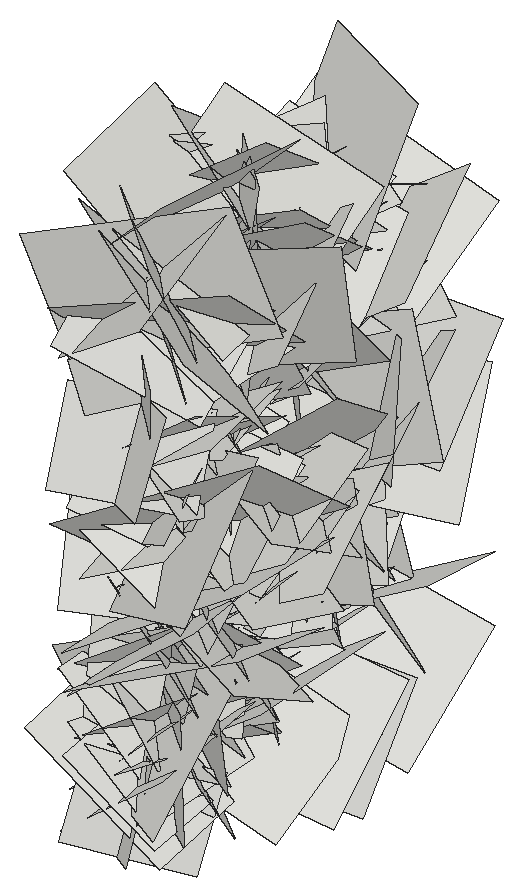
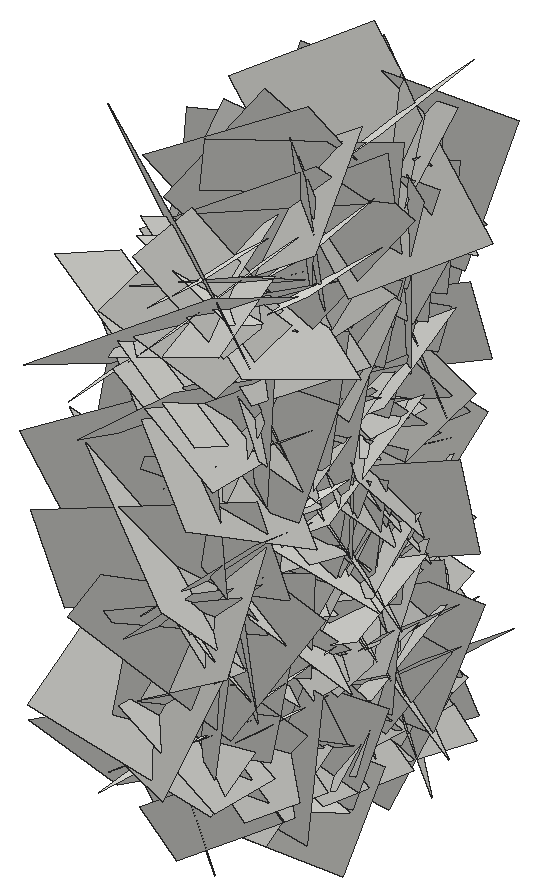
# SketchUp Ruby script. Lengths in inches.
U = 1.inch
M = Sketchup.active_model
def pt(a) = Geom::Point3d.new(a.map { |v| v * U })
def face(e, loops, mat)
  f = e.add_face(loops[0].map { |a| pt(a) })
  loops[1..].each { |l| e.add_face(l.map { |a| pt(a) }).erase! }
  f.material = f.back_material = mat if mat
  f
end
# faces: each face lists its corners as indices into pts; further lists are holes
def faces(e, pts, list, mat = nil) = list.each { |f| face(e, (f[0].is_a?(Array) ? f : [f]).map { |l| l.map { |i| pts[i] } }, mat) }
# xy, xz, yz: faces in a plane at the given z, y or x. An outline is a flat list of corners, or four numbers for a rectangle; further outlines are holes
def ring(l) = l.size == 4 ? [[l[0], l[1]], [l[2], l[1]], [l[2], l[3]], [l[0], l[3]]] : l.each_slice(2).to_a
def flat(e, list, mat, &to3) = list.each { |f| face(e, (f[0].is_a?(Array) ? f : [f]).map { |l| ring(l).map { |u, v| to3.(u, v) } }, mat) }
def xy(e, z, list, mat = nil) = flat(e, list, mat) { |x, y| [x, y, z] }
def xz(e, y, list, mat = nil) = flat(e, list, mat) { |x, z| [x, y, z] }
def yz(e, x, list, mat = nil) = flat(e, list, mat) { |y, z| [x, y, z] }
def lines(e, pts, list) = list.each { |a, b| e.add_line(pt(pts[a]), pt(pts[b])) }
# prism: a flat outline (further loops are holes) pulled along v
def prism(e, loops, v, mat = nil)
  f = face(e, loops, mat); d = Geom::Vector3d.new(v.map { |x| x * U })
  f.pushpull(f.normal.samedirection?(d) ? d.length : -d.length)
end
def box(e, o, s, mat = nil) = prism(e, [[o, [o[0] + s[0], o[1], o[2]], [o[0] + s[0], o[1] + s[1], o[2]], [o[0], o[1] + s[1], o[2]]]], [0, 0, s[2]], mat)
def at(x, y, z, deg = 0) = Geom::Transformation.translation(pt([x, y, z])) * Geom::Transformation.rotation(ORIGIN, Z_AXIS, deg.degrees)
def axes(o, x, y, z) = Geom::Transformation.new([*x, 0, *y, 0, *z, 0, *pt(o).to_a, 1])
def part(name) = M.definitions.add(name)
# library, detail: a bought-in or finely detailed component or shape, given as its bounding box
def library(name, o, s) = part(name).tap { |d| box(d.entities, o, s) }
def detail(e, o, s) = box(e.add_group.entities, o, s)
def put(e, d, t, mat = nil) = e.add_instance(d, t).tap { |i| i.material = mat if mat }
def group(e, t, mat = nil) = e.add_group.tap { |g| g.transformation = t; g.material = mat if mat }.entities
root = M.entities
c1 = part("Component\#6")
p = [[0.01,0,0],[0,3.24,4.54],[4.32,3.24,4.54],[4.33,0,0]]
faces(c1.entities,p,[[0,1,2,3]])
put(root,c1,axes([34.14,187.98,11.49],[-0.12716,0.81746,0.20835],[-0.15,0.18797,-0.81896],[0.88154,0.1499,-0.10929]))
put(root,c1,axes([34.14,186.0625,6.1],[-0.08854,0.52684,0.45627],[0.00383,0.45985,-0.53032],[0.73876,0.06076,0.05744]))
put(root,c1,axes([38.11,181.29,16.68],[-0.08133,-0.245,0.96212],[0.05676,0.96256,0.24939],[-1.05086,0.07095,-0.06099]))
put(root,c1,axes([38.11,184.19,13.53],[-0.08078,-0.49886,0.79857],[-0.01528,0.8017,0.49945],[-0.99796,0.02811,-0.07229]))
put(root,c1,axes([38.11,187.61,11.62],[0.28203,-0.58282,-1.12773],[-0.01249,-1.15332,0.59327],[-1.34554,-0.11146,-0.24188]))
put(root,c1,axes([34.14,183.1,18.89],[-0.1435,0.17311,-0.85276],[-0.14536,-0.85648,-0.1521],[0.91084,-0.10941,-0.15862]))
put(root,c1,axes([34.14,183.83,7.3125],[-0.02805,0.62389,-0.09529],[0.05665,-0.09282,-0.62253],[0.66659,0.03414,0.0489]))
put(root,c1,axes([38.11,184.51,1.15],[0.01173,-1.06899,-0.22188],[0.10644,-0.21996,1.06472],[-1.15237,-0.0312,0.09608]))
put(root,c1,axes([38.11,186.9375,3.03],[-0.11563,0.62873,-0.58509],[-0.05581,-0.59358,-0.62803],[-0.90867,-0.04354,0.11303]))
put(root,c1,axes([34.14,189.45,1.42],[0.1039,0.30381,0.53974],[-0.07033,0.54846,-0.29667],[0.65275,0.01074,-0.11787]))
put(root,c1,axes([34.14,184.54,3.47],[-0.05739,0.5962,-0.42459],[-0.0201,-0.42675,-0.59681],[0.77559,0.03305,-0.04688]))
put(root,c1,axes([38.11,185.64,19.96],[0.2349,1.07139,0.39402],[-0.08081,0.41437,-1.08385],[-1.20734,0.18072,0.1492]))
put(root,c1,axes([38.11,186.72,4.72],[0.08241,-0.91883,0.29273],[-0.13826,0.28096,0.91654],[-1.0128,-0.11312,-0.1013]))
put(root,c1,axes([38.11,190.33,17.67],[-0.17424,0.82504,0.17436],[0.04616,0.18571,-0.83769],[-0.89267,-0.15144,-0.07735]))
put(root,c1,axes([38.11,179.97,24.47],[0.23304,1.36821,0.06434],[0.25904,0.02493,-1.36533],[-1.42861,0.2277,-0.23708]))
put(root,c1,axes([34.14,184.43,15.42],[-0.12844,-0.04329,0.74472],[0.08874,0.74892,0.05716],[0.78574,-0.09166,0.11528]))
put(root,c1,axes([38.11,189.57,16.9],[-0.06471,0.53395,-0.71324],[-0.01751,-0.71546,-0.53421],[-0.94426,-0.02333,0.05878]))
put(root,c1,axes([38.11,191,16.96],[0.17643,-1.14926,-0.11809],[0.05518,-0.11173,1.16072],[-1.22339,-0.17078,0.03532]))
put(root,c1,axes([34.14,186.92,8.78],[-0.10246,-0.30095,0.75916],[-0.04625,0.76527,0.29782],[0.86439,0.00528,0.10592]))
put(root,c1,axes([38.11,180.14,11.99],[0.0212,0.75168,0.8023],[0.17372,0.79143,-0.74558],[-1.15236,0.13314,-0.09764]))
put(root,c1,axes([38.11,185.08,2.16],[-0.06404,-1.02262,-0.11109],[0.17979,-0.11966,1.00929],[-1.07543,0.04089,0.17535]))
put(root,c1,axes([38.11,187.17,12.95],[0.05814,-0.16279,1.09674],[0.14666,1.09051,0.15494],[-1.1661,0.12904,0.07417]))
put(root,c1,axes([38.11,187.85,22.99],[-0.09057,-0.06637,-0.91857],[0.07612,-0.92019,0.05981],[-0.97325,-0.06579,0.09016]))
put(root,c1,axes([34.14,183.375,2.21],[0.01982,-0.33114,-0.74136],[-0.16849,-0.7287,0.32148],[0.84401,-0.13769,0.08159]))
put(root,c1,axes([34.14,192.83,7.86],[0.1126,-0.65912,-0.17655],[-0.1088,-0.19208,0.65534],[0.71507,0.07456,0.12751]))
put(root,c1,axes([38.11,183.46,7.83],[0.1867,0.36795,-0.96583],[-0.13041,-0.96532,-0.39019],[-1.08777,0.17888,-0.11899]))
put(root,c1,axes([38.11,186.63,-0.64],[0.14781,-0.37723,1.01914],[0.01271,1.02797,0.37886],[-1.15185,-0.03706,0.13496]))
put(root,c1,axes([38.11,183.61,1.59],[-0.06331,-0.78644,0.46242],[0.03597,0.46118,0.7887],[-0.96639,0.06869,-0.00094]))
put(root,c1,axes([38.11,185.25,15.47],[-0.04372,0.77316,0.71524],[0.20224,0.70943,-0.75587],[-1.09798,0.09988,-0.16771]))
put(root,c1,axes([38.11,185.13,2.21],[-0.09174,0.69928,0.36],[-0.10121,0.35015,-0.7031],[-0.82753,-0.12035,0.04608]))
put(root,c1,axes([34.14,192.38,19.24],[0.04943,-0.7355,0.057],[-0.07325,0.05251,0.73407],[0.77853,0.05163,0.06545]))
put(root,c1,axes([38.11,181.6,11.88],[-0.05183,0.72565,0.67247],[0.15864,0.67097,-0.71314],[-1.03662,0.0664,-0.14276]))
put(root,c1,axes([34.14,185.26,12.26],[-0.159,0.84642,0.10737],[0.04855,0.11685,-0.85715],[0.9031,0.14274,0.06498]))
put(root,c1,axes([34.14,185.94,13.1875],[-0.12339,0.16979,-0.82402],[0.01755,-0.83125,-0.17361],[0.89164,0.03986,-0.11061]))
put(root,c1,axes([34.14,183.19,13.8],[-0.02762,0.65605,0.3231],[0.06014,0.32414,-0.6536],[0.77284,-0.00178,0.06241]))
put(root,c1,axes([38.11,184.53,11.29],[0.10396,-0.95246,0.37472],[0.04499,0.37989,0.95451],[-1.084,-0.07558,0.07555]))
put(root,c1,axes([38.11,192.08,20.31],[-0.05296,-0.67773,-0.30339],[-0.1724,-0.2867,0.66724],[-0.76797,0.11109,-0.12886]))
put(root,c1,axes([34.14,192.03,8.33],[-0.03388,0.22508,-0.86549],[-0.13142,-0.8588,-0.21876],[0.93879,-0.1121,-0.06186]))
put(root,c1,axes([34.14,185.14,8.49],[0.08576,-0.66072,-0.04627],[0.0456,-0.04128,0.66459],[0.70059,0.08356,-0.03759]))
put(root,c1,axes([34.14,183.28,17.73],[-0.09647,-0.26045,0.74001],[0.11879,0.73302,0.27177],[0.82305,-0.13632,0.04751]))
put(root,c1,axes([34.14,193.37,9.31],[-0.05697,-0.46717,-0.61186],[0.09106,-0.61316,0.46062],[0.81091,0.03603,-0.09471]))
put(root,c1,axes([34.14,191.46,9.82],[-0.08538,-0.06629,-0.92063],[-0.09555,-0.91915,0.07407],[0.97372,-0.09601,-0.07345]))
put(root,c1,axes([34.14,191.35,2.27],[-0.06694,-0.86655,-0.10749],[-0.04783,-0.10439,0.86806],[0.92435,-0.06816,0.03713]))
put(root,c1,axes([34.14,190.84,12.42],[0.00848,-0.77925,-0.15089],[-0.03038,-0.15108,0.77873],[0.8408,0.0024,0.02966]))
put(root,c1,axes([34.14,182.98,9.92],[0.09782,-0.62966,-0.10425],[0.08997,-0.09229,0.63256],[0.67052,0.10424,-0.06967]))
put(root,c1,axes([34.14,180.19,4.07],[0.08532,0.68038,-0.07405],[0.04058,-0.07892,-0.68351],[0.72433,-0.07573,0.04702]))
put(root,c1,axes([34.14,183.91,5.17],[-0.1157,0.58195,-0.7538],[-0.08085,-0.76164,-0.57696],[1.0062,0.00571,-0.13304]))
put(root,c1,axes([34.14,182.875,15.8],[-0.04284,-0.30855,-0.78276],[-0.017,-0.78324,0.30957],[0.8917,-0.02976,-0.0317]))
put(root,c1,axes([38.11,184.33,2.33],[0.23495,-0.78095,0.69461],[-0.033,0.70481,0.80235],[-1.10738,-0.18669,0.12346]))
put(root,c1,axes([38.11,189.86,21.06],[0.09411,0.75469,-0.30292],[-0.23058,-0.27158,-0.74036],[-0.83059,0.16091,0.17121]))
put(root,c1,axes([38.11,189.65,5.54],[-0.06955,0.77959,0.08211],[-0.00823,0.08175,-0.78235],[-0.8309,-0.06607,0.00087]))
put(root,c1,axes([38.11,192.04,5.47],[0.24252,-0.79203,0.72828],[0.0092,0.7459,0.80846],[-1.14049,-0.1624,0.16139]))
put(root,c1,axes([38.11,184.16,21.8125],[0.07155,0.99261,-0.10082],[0.11355,-0.10768,-0.9884],[-1.05147,0.05592,-0.1136]))
put(root,c1,axes([34.14,184.68,7.1],[-0.07537,-0.21143,-0.85755],[-0.01444,-0.85996,0.21315],[0.93612,-0.03029,-0.06575]))
put(root,c1,axes([34.14,187.95,18.35],[-0.24952,-0.85217,0.60628],[-0.01294,0.62364,0.87183],[1.1085,-0.18454,0.14665]))
put(root,c1,axes([38.11,188.38,23.95],[0.14683,-0.05211,-1.06804],[0.1506,-1.06652,0.07046],[-1.12342,-0.14978,-0.13015]))
put(root,c1,axes([34.14,188.38,23.95],[-0.14683,-0.05211,-1.06804],[-0.1506,-1.06652,0.07046],[1.12342,-0.14978,-0.13015]))
put(root,c1,axes([38.11,187.95,18.35],[0.24952,-0.85217,0.60628],[0.01294,0.62364,0.87183],[-1.1085,-0.18454,0.14665]))
put(root,c1,axes([38.11,184.68,7.1],[0.07537,-0.21143,-0.85755],[0.01444,-0.85996,0.21315],[-0.93612,-0.03029,-0.06575]))
put(root,c1,axes([34.14,184.16,21.8125],[-0.07155,0.99261,-0.10082],[-0.11355,-0.10768,-0.9884],[1.05147,0.05592,-0.1136]))
put(root,c1,axes([34.14,192.04,5.47],[-0.24252,-0.79203,0.72828],[-0.0092,0.7459,0.80846],[1.14049,-0.1624,0.16139]))
put(root,c1,axes([34.14,189.65,5.54],[0.06955,0.77959,0.08211],[0.00823,0.08175,-0.78235],[0.8309,-0.06607,0.00087]))
put(root,c1,axes([34.14,189.86,21.06],[-0.09411,0.75469,-0.30292],[0.23058,-0.27158,-0.74036],[0.83059,0.16091,0.17121]))
put(root,c1,axes([34.14,184.33,2.33],[-0.23495,-0.78095,0.69461],[0.033,0.70481,0.80235],[1.10738,-0.18669,0.12346]))
put(root,c1,axes([38.11,182.875,15.8],[0.04284,-0.30855,-0.78276],[0.017,-0.78324,0.30957],[-0.8917,-0.02976,-0.0317]))
put(root,c1,axes([38.11,183.91,5.17],[0.1157,0.58195,-0.7538],[0.08085,-0.76164,-0.57696],[-1.0062,0.00571,-0.13304]))
put(root,c1,axes([38.11,180.19,4.07],[-0.08532,0.68038,-0.07405],[-0.04058,-0.07892,-0.68351],[-0.72433,-0.07573,0.04702]))
put(root,c1,axes([38.11,182.98,9.92],[-0.09782,-0.62966,-0.10425],[-0.08997,-0.09229,0.63256],[-0.67052,0.10424,-0.06967]))
put(root,c1,axes([38.11,190.84,12.42],[-0.00848,-0.77925,-0.15089],[0.03038,-0.15108,0.77873],[-0.8408,0.0024,0.02966]))
put(root,c1,axes([38.11,191.35,2.27],[0.06694,-0.86655,-0.10749],[0.04783,-0.10439,0.86806],[-0.92435,-0.06816,0.03713]))
put(root,c1,axes([38.11,191.46,9.82],[0.08538,-0.06629,-0.92063],[0.09555,-0.91915,0.07407],[-0.97372,-0.09601,-0.07345]))
put(root,c1,axes([38.11,193.37,9.31],[0.05697,-0.46717,-0.61186],[-0.09106,-0.61316,0.46062],[-0.81091,0.03603,-0.09471]))
put(root,c1,axes([38.11,183.28,17.73],[0.09647,-0.26045,0.74001],[-0.11879,0.73302,0.27177],[-0.82305,-0.13632,0.04751]))
put(root,c1,axes([38.11,185.14,8.49],[-0.08576,-0.66072,-0.04627],[-0.0456,-0.04128,0.66459],[-0.70059,0.08356,-0.03759]))
put(root,c1,axes([38.11,192.03,8.33],[0.03388,0.22508,-0.86549],[0.13142,-0.8588,-0.21876],[-0.93879,-0.1121,-0.06186]))
put(root,c1,axes([34.14,192.08,20.31],[0.05296,-0.67773,-0.30339],[0.1724,-0.2867,0.66724],[0.76797,0.11109,-0.12886]))
put(root,c1,axes([34.14,184.53,11.29],[-0.10396,-0.95246,0.37472],[-0.04499,0.37989,0.95451],[1.084,-0.07558,0.07555]))
put(root,c1,axes([38.11,183.19,13.8],[0.02762,0.65605,0.3231],[-0.06014,0.32414,-0.6536],[-0.77284,-0.00178,0.06241]))
put(root,c1,axes([38.11,185.94,13.1875],[0.12339,0.16979,-0.82402],[-0.01755,-0.83125,-0.17361],[-0.89164,0.03986,-0.11061]))
put(root,c1,axes([38.11,185.26,12.26],[0.159,0.84642,0.10737],[-0.04855,0.11685,-0.85715],[-0.9031,0.14274,0.06498]))
put(root,c1,axes([34.14,181.6,11.88],[0.05183,0.72565,0.67247],[-0.15864,0.67097,-0.71314],[1.03662,0.0664,-0.14276]))
put(root,c1,axes([38.11,192.38,19.24],[-0.04943,-0.7355,0.057],[0.07325,0.05251,0.73407],[-0.77853,0.05163,0.06545]))
put(root,c1,axes([34.14,185.13,2.21],[0.09174,0.69928,0.36],[0.10121,0.35015,-0.7031],[0.82753,-0.12035,0.04608]))
put(root,c1,axes([34.14,185.25,15.47],[0.04372,0.77316,0.71524],[-0.20224,0.70943,-0.75587],[1.09798,0.09988,-0.16771]))
put(root,c1,axes([34.14,183.61,1.59],[0.06331,-0.78644,0.46242],[-0.03597,0.46118,0.7887],[0.96639,0.06869,-0.00094]))
put(root,c1,axes([34.14,186.63,-0.64],[-0.14781,-0.37723,1.01914],[-0.01271,1.02797,0.37886],[1.15185,-0.03706,0.13496]))
put(root,c1,axes([34.14,183.46,7.83],[-0.1867,0.36795,-0.96583],[0.13041,-0.96532,-0.39019],[1.08777,0.17888,-0.11899]))
put(root,c1,axes([38.11,192.83,7.86],[-0.1126,-0.65912,-0.17655],[0.1088,-0.19208,0.65534],[-0.71507,0.07456,0.12751]))
put(root,c1,axes([38.11,183.375,2.21],[-0.01982,-0.33114,-0.74136],[0.16849,-0.7287,0.32148],[-0.84401,-0.13769,0.08159]))
put(root,c1,axes([34.14,187.85,22.99],[0.09057,-0.06637,-0.91857],[-0.07612,-0.92019,0.05981],[0.97325,-0.06579,0.09016]))
put(root,c1,axes([34.14,187.17,12.95],[-0.05814,-0.16279,1.09674],[-0.14666,1.09051,0.15494],[1.1661,0.12904,0.07417]))
put(root,c1,axes([34.14,185.08,2.16],[0.06404,-1.02262,-0.11109],[-0.17979,-0.11966,1.00929],[1.07543,0.04089,0.17535]))
put(root,c1,axes([34.14,180.14,11.99],[-0.0212,0.75168,0.8023],[-0.17372,0.79143,-0.74558],[1.15236,0.13314,-0.09764]))
put(root,c1,axes([38.11,186.92,8.78],[0.10246,-0.30095,0.75916],[0.04625,0.76527,0.29782],[-0.86439,0.00528,0.10592]))
put(root,c1,axes([34.14,191,16.96],[-0.17643,-1.14926,-0.11809],[-0.05518,-0.11173,1.16072],[1.22339,-0.17078,0.03532]))
put(root,c1,axes([34.14,189.57,16.9],[0.06471,0.53395,-0.71324],[0.01751,-0.71546,-0.53421],[0.94426,-0.02333,0.05878]))
put(root,c1,axes([38.11,184.43,15.42],[0.12844,-0.04329,0.74472],[-0.08874,0.74892,0.05716],[-0.78574,-0.09166,0.11528]))
put(root,c1,axes([34.14,179.97,24.47],[-0.23304,1.36821,0.06434],[-0.25904,0.02493,-1.36533],[1.42861,0.2277,-0.23708]))
put(root,c1,axes([38.11,182.67,1.51],[0.02969,-0.72745,-0.10184],[0.03667,-0.1005,0.72735],[-0.77775,-0.03251,0.03041]))
put(root,c1,axes([34.14,190.33,17.67],[0.17424,0.82504,0.17436],[-0.04616,0.18571,-0.83769],[0.89267,-0.15144,-0.07735]))
put(root,c1,axes([34.14,186.72,4.72],[-0.08241,-0.91883,0.29273],[0.13826,0.28096,0.91654],[1.0128,-0.11312,-0.1013]))
put(root,c1,axes([34.14,185.64,19.96],[-0.2349,1.07139,0.39402],[0.08081,0.41437,-1.08385],[1.20734,0.18072,0.1492]))
put(root,c1,axes([38.11,184.54,3.47],[0.05739,0.5962,-0.42459],[0.0201,-0.42675,-0.59681],[-0.77559,0.03305,-0.04688]))
put(root,c1,axes([38.11,189.45,1.42],[-0.1039,0.30381,0.53974],[0.07033,0.54846,-0.29667],[-0.65275,0.01074,-0.11787]))
put(root,c1,axes([34.14,186.9375,3.03],[0.11563,0.62873,-0.58509],[0.05581,-0.59358,-0.62803],[0.90867,-0.04354,0.11303]))
put(root,c1,axes([34.14,184.51,1.15],[-0.01173,-1.06899,-0.22188],[-0.10644,-0.21996,1.06472],[1.15237,-0.0312,0.09608]))
put(root,c1,axes([38.11,183.83,7.3125],[0.02805,0.62389,-0.09529],[-0.05665,-0.09282,-0.62253],[-0.66659,0.03414,0.0489]))
put(root,c1,axes([38.11,183.1,18.89],[0.1435,0.17311,-0.85276],[0.14536,-0.85648,-0.1521],[-0.91084,-0.10941,-0.15862]))
put(root,c1,axes([34.14,187.61,11.62],[-0.28203,-0.58282,-1.12773],[0.01249,-1.15332,0.59327],[1.34554,-0.11146,-0.24188]))
put(root,c1,axes([34.14,184.19,13.53],[0.08078,-0.49886,0.79857],[0.01528,0.8017,0.49945],[0.99796,0.02811,-0.07229]))
put(root,c1,axes([34.14,181.29,16.68],[0.08133,-0.245,0.96212],[-0.05676,0.96256,0.24939],[1.05086,0.07095,-0.06099]))
put(root,c1,axes([38.11,186.0625,6.1],[0.08854,0.52684,0.45627],[-0.00383,0.45985,-0.53032],[-0.73876,0.06076,0.05744]))
put(root,c1,axes([38.11,187.98,11.49],[0.12716,0.81746,0.20835],[0.15,0.18797,-0.81896],[-0.88154,0.1499,-0.10929]))
put(root,c1,axes([34.14,194.3,13.93],[-0.22437,-1.23478,-0.60854],[-0.19245,-0.58527,1.25072],[1.44644,-0.26941,0.07201]))
put(root,c1,axes([34.14,184.41,20.14],[-0.03821,-1.03167,-0.60174],[-0.15497,-0.59368,1.0266],[1.25647,-0.1046,0.10832]))
put(root,c1,axes([38.11,186.3,8.38],[-0.07617,0.47932,0.41871],[0.13681,0.42359,-0.46276],[-0.66062,0.03245,-0.14411]))
put(root,c1,axes([34.14,184.31,4.6],[0.1576,-0.1516,-1.0147],[-0.15202,-1.0183,0.13112],[1.07684,-0.12157,0.16702]))
put(root,c1,axes([34.14,179.32,18.3],[0.15069,0.54422,0.74866],[-0.00735,0.75804,-0.54972],[0.98107,-0.07791,-0.11911]))
put(root,c1,axes([38.11,188.8,6.44],[0.14743,-0.18272,-0.74199],[0.06403,-0.74919,0.19581],[-0.80747,-0.09277,-0.11994]))
put(root,c1,axes([34.14,185.52,6.2],[-0.2751,-0.65276,-1.16933],[-0.03559,-1.18754,0.67037],[1.41909,-0.15632,-0.20987]))
put(root,c1,axes([34.14,181.08,20.02],[-0.00536,1.00575,0.03656],[0.10796,0.03689,-1.00058],[1.06133,0.00133,0.10197]))
put(root,c1,axes([34.14,184.05,20.67],[0.10102,0.73684,0.6989],[-0.04073,0.70408,-0.73707],[1.07574,-0.04254,-0.09354]))
put(root,c1,axes([34.14,191.125,9.45],[-0.23474,-0.88576,-0.93612],[0.00151,-0.95001,0.89856],[1.36608,-0.15116,-0.16185]))
put(root,c1,axes([34.14,185.11,13.22],[0.08906,-0.95701,-0.12674],[0.0585,-0.12225,0.95969],[1.02162,0.09043,-0.0439]))
put(root,c1,axes([34.14,180.4,17.125],[-0.23878,-0.31981,1.17522],[0.15258,1.17979,0.34864],[1.28199,-0.19998,0.17739]))
put(root,c1,axes([34.14,187.48,17.59],[-0.04794,-0.78864,0.66349],[0.19289,0.64758,0.78214],[1.07529,-0.15133,-0.11072]))
put(root,c1,axes([34.14,187.26,9.21],[0.06299,-0.71122,-0.64775],[0.16214,-0.63375,0.70987],[1.00673,0.14657,-0.0738]))
put(root,c1,axes([38.11,191.11,1.26],[0.04561,-0.57908,-0.31344],[0.1156,-0.3035,0.57569],[-0.68833,-0.08935,0.07592]))
put(root,c1,axes([34.14,186.13,19.34],[0.13168,0.96657,0.23982],[0.01085,0.24043,-0.97432],[1.05558,-0.12304,-0.0199]))
put(root,c1,axes([34.14,188.68,19.83],[-0.08458,1.11358,0.50301],[-0.01593,0.50315,-1.11627],[1.29513,0.07891,0.01912]))
put(root,c1,axes([34.14,185.36,5.79],[0.02078,-1.22604,-0.15411],[-0.11589,-0.15525,1.22117],[1.3047,0.00574,0.11093]))
put(root,c1,axes([34.14,186.43,6.6],[-0.00451,1.27416,-0.10814],[-0.14001,-0.108,-1.26731],[1.34821,-0.00695,-0.13197]))
put(root,c1,axes([38.11,190.35,18.26],[0.16101,-0.65287,0.16772],[0.08445,0.18811,0.66008],[-0.7095,-0.12576,0.11663]))
put(root,c1,axes([34.14,187.9375,5.11],[0.04973,-1.23753,-0.07043],[-0.13139,-0.07481,1.23194],[1.30732,0.03956,0.12649]))
put(root,c1,axes([34.14,189.08,9.2],[-0.13088,0.55221,1.09741],[0.12619,1.10312,-0.54169],[1.29609,-0.05164,0.16356]))
put(root,c1,axes([34.14,182.44,13.63],[-0.1579,1.28482,-0.45217],[-0.02165,-0.45692,-1.2916],[1.44363,0.13368,-0.06883]))
put(root,c1,axes([34.14,182.53,23.48],[0.24403,0.37129,-0.99391],[-0.1038,-1.00526,-0.39821],[1.11985,-0.17408,0.17968]))
put(root,c1,axes([34.14,192.17,8.01],[0.17438,0.53527,-0.89237],[0.02164,-0.90494,-0.53904],[1.10282,-0.06688,0.15168]))
put(root,c1,axes([34.14,188.23,7.57],[0.0913,-1.12353,0.75234],[-0.27462,0.72618,1.11413],[1.40673,0.21468,0.16867]))
put(root,c1,axes([34.14,194.04,23.84],[-0.15699,-0.54259,-1.24113],[0.03696,-1.24964,0.54215],[1.43535,-0.02717,-0.14971]))
put(root,c1,axes([34.14,189.36,1.43],[-0.09807,-1.35815,-0.14277],[-0.05055,-0.1398,1.36078],[1.44669,-0.09695,0.03787]))
put(root,c1,axes([34.14,188.7,21.97],[0.14471,1.28216,-0.28655],[-0.25359,-0.25902,-1.27293],[1.36933,-0.18346,-0.20546]))
put(root,c1,axes([34.14,190.12,11.53],[-0.21117,-0.99907,-0.90649],[0.1512,-0.92678,0.99009],[1.42194,-0.04983,-0.2399]))
put(root,c1,axes([34.14,183.02,16.38],[-0.02893,-0.8566,0.75588],[0.26219,0.73373,0.84043],[1.18223,-0.18368,-0.16789]))
put(root,c1,axes([34.14,185.31,6.45],[-0.03902,-0.20515,1.15818],[0.22164,1.13915,0.20842],[1.22693,-0.21231,-0.00082]))
put(root,c1,axes([34.14,180.93,10.86],[-0.17521,1.15715,-0.62152],[0.20897,-0.59747,-1.1648],[1.37654,0.23798,0.09772]))
put(root,c1,axes([34.14,184.5,10.44],[0.20009,0.552,-0.98447],[-0.02572,-0.99592,-0.56307],[1.1961,-0.11375,0.15258]))
put(root,c1,axes([34.14,185.25,0.97],[0.15144,0.45294,1.0525],[0.02813,1.05906,-0.45936],[1.21425,-0.08102,-0.12063]))
put(root,c1,axes([34.14,182.38,2.76],[0.16715,0.82367,0.72398],[0.09449,0.71938,-0.83785],[1.15857,-0.1775,-0.03612]))
put(root,c1,axes([34.14,186.66,10.07],[-0.09303,-0.2424,1.37134],[-0.00293,1.37409,0.24271],[1.47615,-0.01254,0.08691]))
put(root,c1,axes([34.14,192.77,15.58],[0.03721,-0.16955,-1.17702],[0.1418,-1.1695,0.17246],[1.25252,0.13744,0.01545]))
put(root,c1,axes([34.14,185.87,11.99],[0.00632,-0.88407,-1.06115],[-0.10628,-1.05864,0.88141],[1.46017,-0.07323,0.06874]))
put(root,c1,axes([34.14,186.02,17.55],[0.12484,-0.91824,0.67786],[0.09261,0.68671,0.91505],[1.20627,0.04231,-0.14041]))
put(root,c1,axes([34.14,195.54,11.625],[0.04246,-1.00606,-0.92627],[-0.11693,-0.92602,1.00103],[1.44486,-0.04538,0.10823]))
put(root,c1,axes([34.14,183.88,15.08],[-0.0404,1.11797,-0.62329],[0.16276,-0.61507,-1.11262],[1.34698,0.10785,0.11575]))
put(root,c1,axes([34.14,184.23,21.55],[0.30098,0.54789,0.85036],[0.10123,0.86476,-0.58905],[1.06749,-0.23649,-0.1839]))
put(root,c1,axes([34.14,184,8.18],[-0.02134,-1.06466,0.81449],[0.04088,0.81378,1.06469],[1.42032,-0.03942,-0.01841]))
put(root,c1,axes([34.14,188.34,12.62],[0.20954,0.481,1.15591],[-0.07101,1.17261,-0.47649],[1.32521,-0.01322,-0.2083]))
put(root,c1,axes([34.14,186.39,13.5625],[0.22643,-0.80881,0.81079],[0.0736,0.83241,0.81208],[1.21171,0.10058,-0.20084]))
put(root,c1,axes([34.14,184.34,4.6],[0.11485,-1.15497,0.26483],[0.19184,0.27894,1.14248],[1.2413,0.06375,-0.20107]))
put(root,c1,axes([34.14,193.03,3.2],[0.23388,-1.096,0.27231],[0.13541,0.2999,1.10354],[1.1894,0.18138,-0.17918]))
put(root,c1,axes([34.14,189.55,17.94],[0.16397,-1.09761,-0.83604],[-0.11999,-0.84854,1.09307],[1.45761,0.05363,0.18403]))
put(root,c1,axes([34.14,187.39,3.1875],[0.10139,0.89849,0.89189],[0.1671,0.87902,-0.90243],[1.33152,-0.17873,0.04534]))
put(root,c1,axes([34.14,180.76,23.09],[0.06995,0.91309,-0.96842],[0.10566,-0.97028,-0.90805],[1.4069,0.02747,0.11634]))
put(root,c1,axes([34.14,183.54,2.14],[0.03864,0.84179,0.92004],[0.33491,0.88417,-0.82148],[1.27872,-0.257,0.18735]))
put(root,c1,axes([34.14,184.58,6.82],[0.16596,-1.29847,0.14138],[0.0614,0.14916,1.30572],[1.38315,0.14917,-0.07492]))
put(root,c1,axes([34.14,193.85,16.74],[0.30124,-1.14539,-0.57535],[-0.00001,-0.58933,1.17321],[1.35869,0.25394,0.12757]))
put(root,c1,axes([34.14,189.11,8.53],[0.25892,-1.11224,-0.53402],[0.14932,-0.51568,1.13849],[1.29927,0.28091,-0.02442]))
put(root,c1,axes([34.14,182.27,16.13],[0.23771,-0.47409,1.27281],[0.00404,1.29026,0.47991],[1.43973,0.07465,-0.2115]))
